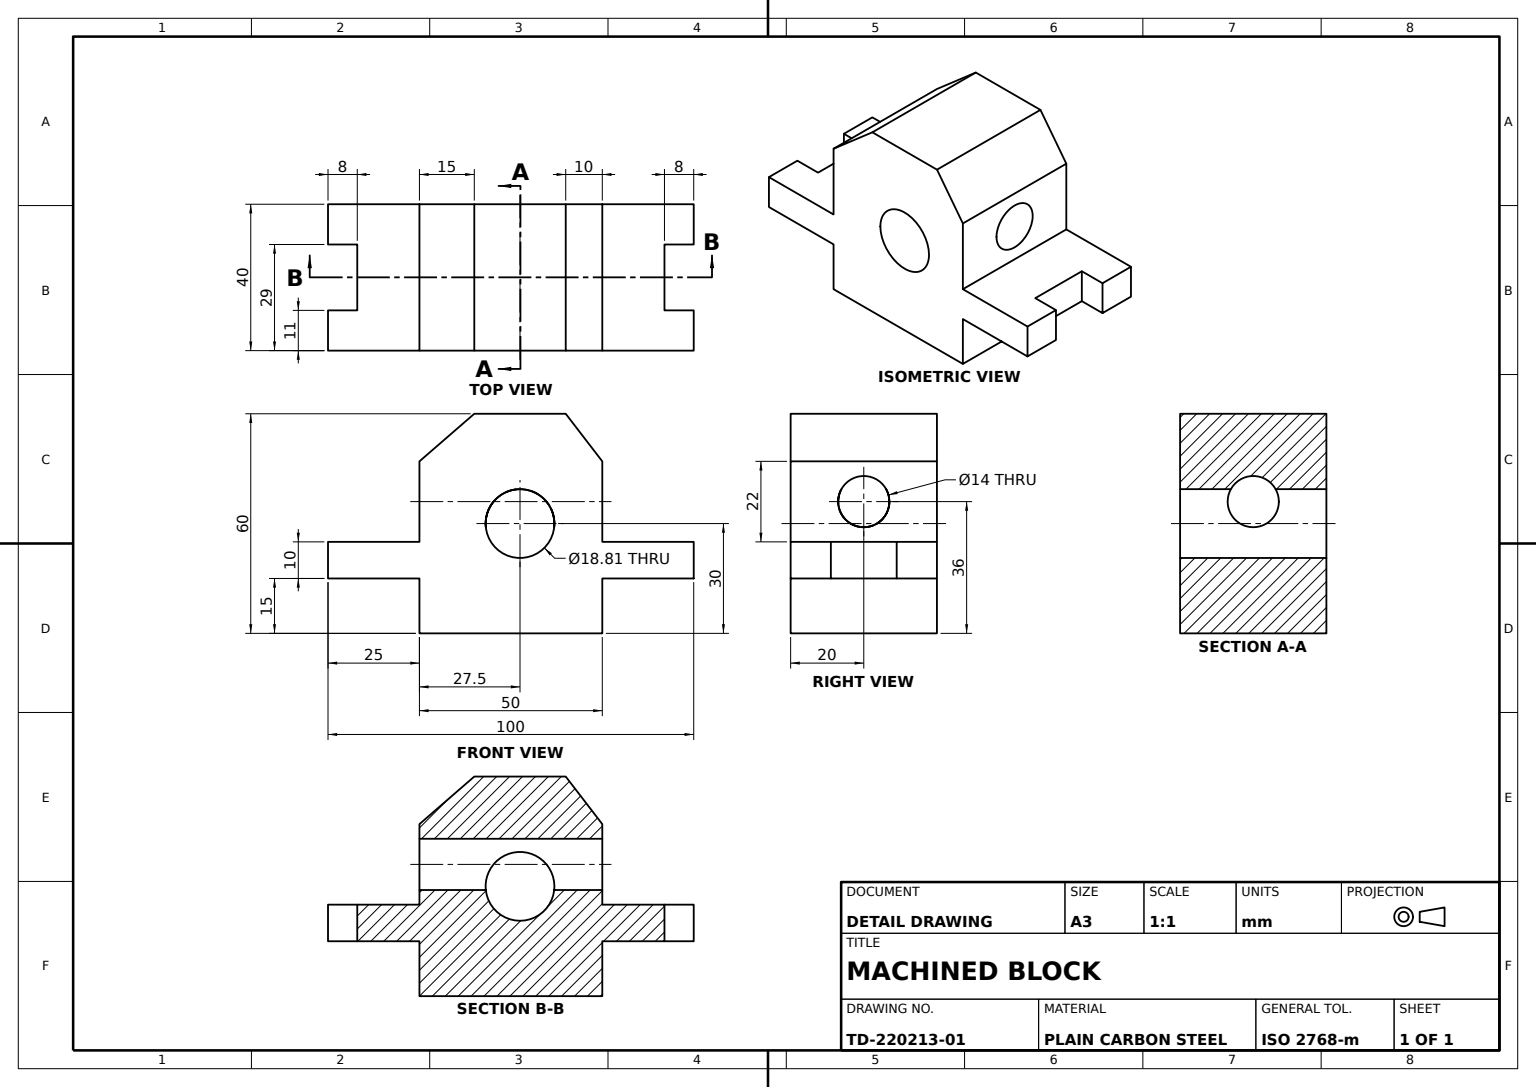
ISO-10303-21;
HEADER;
FILE_DESCRIPTION((''),'2;1');
FILE_NAME('','',(''),(''),'','','');
FILE_SCHEMA(('AUTOMOTIVE_DESIGN'));
ENDSEC;
DATA;
#1=APPLICATION_CONTEXT('');
#2=PRODUCT_CONTEXT('',#1,'mechanical');
#3=PRODUCT('','','',(#2));
#4=PRODUCT_DEFINITION_FORMATION('','',#3);
#5=PRODUCT_DEFINITION_CONTEXT('',#1,'design');
#6=PRODUCT_DEFINITION('','',#4,#5);
#7=PRODUCT_DEFINITION_SHAPE('','',#6);
#8=(LENGTH_UNIT()NAMED_UNIT(*)SI_UNIT(.MILLI.,.METRE.));
#9=(NAMED_UNIT(*)PLANE_ANGLE_UNIT()SI_UNIT($,.RADIAN.));
#10=(NAMED_UNIT(*)SI_UNIT($,.STERADIAN.)SOLID_ANGLE_UNIT());
#11=UNCERTAINTY_MEASURE_WITH_UNIT(LENGTH_MEASURE(1.E-05),#8,'distance_accuracy_value','');
#12=(GEOMETRIC_REPRESENTATION_CONTEXT(3)GLOBAL_UNCERTAINTY_ASSIGNED_CONTEXT((#11))GLOBAL_UNIT_ASSIGNED_CONTEXT((#8,#9,#10))REPRESENTATION_CONTEXT('',''));
#13=CARTESIAN_POINT('',(50.,36.,27.));
#14=VERTEX_POINT('',#13);
#15=CARTESIAN_POINT('',(50.,36.,13.));
#16=VERTEX_POINT('',#15);
#17=CARTESIAN_POINT('',(50.,36.,20.));
#18=DIRECTION('',(1.,0.,0.));
#19=DIRECTION('',(0.,0.,-1.));
#20=AXIS2_PLACEMENT_3D('',#17,#18,#19);
#21=CIRCLE('',#20,7.);
#22=EDGE_CURVE('',#14,#16,#21,.T.);
#23=ORIENTED_EDGE('',*,*,#22,.F.);
#24=EDGE_CURVE('',#16,#14,#21,.T.);
#25=ORIENTED_EDGE('',*,*,#24,.F.);
#26=EDGE_LOOP('',(#23,#25));
#27=FACE_BOUND('',#26,.T.);
#28=CARTESIAN_POINT('',(50.,25.,0.));
#29=VERTEX_POINT('',#28);
#30=CARTESIAN_POINT('',(50.,47.,0.));
#31=VERTEX_POINT('',#30);
#32=DIRECTION('',(0.,1.,0.));
#33=VECTOR('',#32,1000.);
#34=LINE('',#28,#33);
#35=EDGE_CURVE('',#29,#31,#34,.T.);
#36=ORIENTED_EDGE('',*,*,#35,.T.);
#37=CARTESIAN_POINT('',(50.,47.,40.));
#38=VERTEX_POINT('',#37);
#39=VECTOR('',#19,1000.);
#40=LINE('',#37,#39);
#41=EDGE_CURVE('',#38,#31,#40,.T.);
#42=ORIENTED_EDGE('',*,*,#41,.F.);
#43=CARTESIAN_POINT('',(50.,25.,40.));
#44=VERTEX_POINT('',#43);
#45=LINE('',#43,#33);
#46=EDGE_CURVE('',#44,#38,#45,.T.);
#47=ORIENTED_EDGE('',*,*,#46,.F.);
#48=LINE('',#43,#39);
#49=EDGE_CURVE('',#44,#29,#48,.T.);
#50=ORIENTED_EDGE('',*,*,#49,.T.);
#51=EDGE_LOOP('',(#36,#42,#47,#50));
#52=FACE_OUTER_BOUND('',#51,.T.);
#53=DIRECTION('',(-1.,0.,0.));
#54=DIRECTION('',(0.,0.,1.));
#55=AXIS2_PLACEMENT_3D('',#43,#53,#54);
#56=PLANE('',#55);
#57=ADVANCED_FACE('',(#27,#52),#56,.F.);
#58=CARTESIAN_POINT('',(50.,15.,40.));
#59=VERTEX_POINT('',#58);
#60=CARTESIAN_POINT('',(50.,15.,0.));
#61=VERTEX_POINT('',#60);
#62=LINE('',#58,#39);
#63=EDGE_CURVE('',#59,#61,#62,.T.);
#64=ORIENTED_EDGE('',*,*,#63,.F.);
#65=CARTESIAN_POINT('',(50.,0.,40.));
#66=VERTEX_POINT('',#65);
#67=LINE('',#65,#33);
#68=EDGE_CURVE('',#66,#59,#67,.T.);
#69=ORIENTED_EDGE('',*,*,#68,.F.);
#70=CARTESIAN_POINT('',(50.,0.,0.));
#71=VERTEX_POINT('',#70);
#72=LINE('',#65,#39);
#73=EDGE_CURVE('',#66,#71,#72,.T.);
#74=ORIENTED_EDGE('',*,*,#73,.T.);
#75=LINE('',#70,#33);
#76=EDGE_CURVE('',#71,#61,#75,.T.);
#77=ORIENTED_EDGE('',*,*,#76,.T.);
#78=EDGE_LOOP('',(#64,#69,#74,#77));
#79=FACE_OUTER_BOUND('',#78,.T.);
#80=AXIS2_PLACEMENT_3D('',#65,#53,#54);
#81=PLANE('',#80);
#82=ADVANCED_FACE('',(#79),#81,.F.);
#83=CARTESIAN_POINT('',(67.,25.,11.));
#84=VERTEX_POINT('',#83);
#85=CARTESIAN_POINT('',(67.,25.,29.));
#86=VERTEX_POINT('',#85);
#87=VECTOR('',#54,1000.);
#88=LINE('',#83,#87);
#89=EDGE_CURVE('',#84,#86,#88,.T.);
#90=ORIENTED_EDGE('',*,*,#89,.F.);
#91=CARTESIAN_POINT('',(75.,25.,11.));
#92=VERTEX_POINT('',#91);
#93=VECTOR('',#53,1000.);
#94=LINE('',#91,#93);
#95=EDGE_CURVE('',#92,#84,#94,.T.);
#96=ORIENTED_EDGE('',*,*,#95,.F.);
#97=CARTESIAN_POINT('',(75.,25.,0.));
#98=VERTEX_POINT('',#97);
#99=CARTESIAN_POINT('',(75.,25.,40.));
#100=LINE('',#99,#39);
#101=EDGE_CURVE('',#92,#98,#100,.T.);
#102=ORIENTED_EDGE('',*,*,#101,.T.);
#103=LINE('',#97,#93);
#104=EDGE_CURVE('',#98,#29,#103,.T.);
#105=ORIENTED_EDGE('',*,*,#104,.T.);
#106=ORIENTED_EDGE('',*,*,#49,.F.);
#107=VERTEX_POINT('',#99);
#108=LINE('',#99,#93);
#109=EDGE_CURVE('',#107,#44,#108,.T.);
#110=ORIENTED_EDGE('',*,*,#109,.F.);
#111=CARTESIAN_POINT('',(75.,25.,29.));
#112=VERTEX_POINT('',#111);
#113=EDGE_CURVE('',#107,#112,#100,.T.);
#114=ORIENTED_EDGE('',*,*,#113,.T.);
#115=VECTOR('',#18,1000.);
#116=LINE('',#85,#115);
#117=EDGE_CURVE('',#86,#112,#116,.T.);
#118=ORIENTED_EDGE('',*,*,#117,.F.);
#119=EDGE_LOOP('',(#90,#96,#102,#105,#106,#110,#114,#118));
#120=FACE_OUTER_BOUND('',#119,.T.);
#121=DIRECTION('',(0.,-1.,0.));
#122=AXIS2_PLACEMENT_3D('',#99,#121,#19);
#123=PLANE('',#122);
#124=ADVANCED_FACE('',(#120),#123,.F.);
#125=CARTESIAN_POINT('',(75.,15.,29.));
#126=VERTEX_POINT('',#125);
#127=CARTESIAN_POINT('',(75.,-15.,29.));
#128=LINE('',#127,#33);
#129=EDGE_CURVE('',#126,#112,#128,.T.);
#130=ORIENTED_EDGE('',*,*,#129,.T.);
#131=ORIENTED_EDGE('',*,*,#113,.F.);
#132=CARTESIAN_POINT('',(75.,15.,40.));
#133=VERTEX_POINT('',#132);
#134=LINE('',#132,#33);
#135=EDGE_CURVE('',#133,#107,#134,.T.);
#136=ORIENTED_EDGE('',*,*,#135,.F.);
#137=LINE('',#132,#39);
#138=EDGE_CURVE('',#133,#126,#137,.T.);
#139=ORIENTED_EDGE('',*,*,#138,.T.);
#140=EDGE_LOOP('',(#130,#131,#136,#139));
#141=FACE_OUTER_BOUND('',#140,.T.);
#142=AXIS2_PLACEMENT_3D('',#132,#53,#54);
#143=PLANE('',#142);
#144=ADVANCED_FACE('',(#141),#143,.F.);
#145=ORIENTED_EDGE('',*,*,#41,.T.);
#146=CARTESIAN_POINT('',(40.,60.,0.));
#147=VERTEX_POINT('',#146);
#148=DIRECTION('',(0.609710761,-0.792623989,0.));
#149=VECTOR('',#148,1000.);
#150=LINE('',#146,#149);
#151=EDGE_CURVE('',#147,#31,#150,.T.);
#152=ORIENTED_EDGE('',*,*,#151,.F.);
#153=CARTESIAN_POINT('',(40.,60.,40.));
#154=VERTEX_POINT('',#153);
#155=LINE('',#153,#39);
#156=EDGE_CURVE('',#154,#147,#155,.T.);
#157=ORIENTED_EDGE('',*,*,#156,.F.);
#158=LINE('',#153,#149);
#159=EDGE_CURVE('',#154,#38,#158,.T.);
#160=ORIENTED_EDGE('',*,*,#159,.T.);
#161=EDGE_LOOP('',(#145,#152,#157,#160));
#162=FACE_OUTER_BOUND('',#161,.T.);
#163=DIRECTION('',(0.792623989,0.609710761,0.));
#164=DIRECTION('',(-0.609710761,0.792623989,0.));
#165=AXIS2_PLACEMENT_3D('',#153,#163,#164);
#166=PLANE('',#165);
#167=ADVANCED_FACE('',(#162),#166,.T.);
#168=CARTESIAN_POINT('',(0.,36.,27.));
#169=VERTEX_POINT('',#168);
#170=CARTESIAN_POINT('',(0.,36.,13.));
#171=VERTEX_POINT('',#170);
#172=CARTESIAN_POINT('',(0.,36.,20.));
#173=AXIS2_PLACEMENT_3D('',#172,#53,#54);
#174=CIRCLE('',#173,7.);
#175=EDGE_CURVE('',#169,#171,#174,.T.);
#176=ORIENTED_EDGE('',*,*,#175,.F.);
#177=EDGE_CURVE('',#171,#169,#174,.T.);
#178=ORIENTED_EDGE('',*,*,#177,.F.);
#179=EDGE_LOOP('',(#176,#178));
#180=FACE_BOUND('',#179,.T.);
#181=CARTESIAN_POINT('',(0.,25.,0.));
#182=VERTEX_POINT('',#181);
#183=CARTESIAN_POINT('',(0.,47.,0.));
#184=VERTEX_POINT('',#183);
#185=LINE('',#181,#33);
#186=EDGE_CURVE('',#182,#184,#185,.T.);
#187=ORIENTED_EDGE('',*,*,#186,.F.);
#188=CARTESIAN_POINT('',(0.,25.,40.));
#189=VERTEX_POINT('',#188);
#190=LINE('',#188,#39);
#191=EDGE_CURVE('',#189,#182,#190,.T.);
#192=ORIENTED_EDGE('',*,*,#191,.F.);
#193=CARTESIAN_POINT('',(0.,47.,40.));
#194=VERTEX_POINT('',#193);
#195=LINE('',#188,#33);
#196=EDGE_CURVE('',#189,#194,#195,.T.);
#197=ORIENTED_EDGE('',*,*,#196,.T.);
#198=LINE('',#193,#39);
#199=EDGE_CURVE('',#194,#184,#198,.T.);
#200=ORIENTED_EDGE('',*,*,#199,.T.);
#201=EDGE_LOOP('',(#187,#192,#197,#200));
#202=FACE_OUTER_BOUND('',#201,.T.);
#203=AXIS2_PLACEMENT_3D('',#188,#53,#54);
#204=PLANE('',#203);
#205=ADVANCED_FACE('',(#180,#202),#204,.T.);
#206=CARTESIAN_POINT('',(75.,15.,11.));
#207=VERTEX_POINT('',#206);
#208=CARTESIAN_POINT('',(75.,-15.,11.));
#209=LINE('',#208,#33);
#210=EDGE_CURVE('',#207,#92,#209,.T.);
#211=ORIENTED_EDGE('',*,*,#210,.T.);
#212=ORIENTED_EDGE('',*,*,#95,.T.);
#213=CARTESIAN_POINT('',(67.,15.,11.));
#214=VERTEX_POINT('',#213);
#215=CARTESIAN_POINT('',(67.,-15.,11.));
#216=LINE('',#215,#33);
#217=EDGE_CURVE('',#214,#84,#216,.T.);
#218=ORIENTED_EDGE('',*,*,#217,.F.);
#219=CARTESIAN_POINT('',(50.,15.,11.));
#220=LINE('',#219,#93);
#221=EDGE_CURVE('',#207,#214,#220,.T.);
#222=ORIENTED_EDGE('',*,*,#221,.F.);
#223=EDGE_LOOP('',(#211,#212,#218,#222));
#224=FACE_OUTER_BOUND('',#223,.T.);
#225=AXIS2_PLACEMENT_3D('',#208,#19,#53);
#226=PLANE('',#225);
#227=ADVANCED_FACE('',(#224),#226,.F.);
#228=CARTESIAN_POINT('',(36.903768,30.,40.));
#229=VERTEX_POINT('',#228);
#230=CARTESIAN_POINT('',(18.096232,30.,40.));
#231=VERTEX_POINT('',#230);
#232=CARTESIAN_POINT('',(27.5,30.,40.));
#233=AXIS2_PLACEMENT_3D('',#232,#54,#18);
#234=CIRCLE('',#233,9.403768);
#235=EDGE_CURVE('',#229,#231,#234,.T.);
#236=ORIENTED_EDGE('',*,*,#235,.T.);
#237=CARTESIAN_POINT('',(18.096232,30.,23.605551));
#238=VERTEX_POINT('',#237);
#239=CARTESIAN_POINT('',(18.096232,30.,0.));
#240=LINE('',#239,#87);
#241=EDGE_CURVE('',#238,#231,#240,.T.);
#242=ORIENTED_EDGE('',*,*,#241,.F.);
#243=CARTESIAN_POINT('',(20.259084,36.,27.));
#244=VERTEX_POINT('',#243);
#245=CARTESIAN_POINT('',(18.096232,30.33094,24.156269));
#246=CARTESIAN_POINT('',(18.112771,30.730821,24.653008));
#247=CARTESIAN_POINT('',(18.20319,31.43388,25.315471));
#248=CARTESIAN_POINT('',(18.244042,31.681225,25.517877));
#249=CARTESIAN_POINT('',(18.351805,32.193127,25.88273));
#250=CARTESIAN_POINT('',(18.41881,32.458633,26.046052));
#251=CARTESIAN_POINT('',(18.585264,33.00672,26.335321));
#252=CARTESIAN_POINT('',(18.685614,33.290821,26.461416));
#253=CARTESIAN_POINT('',(18.916067,33.852142,26.669052));
#254=CARTESIAN_POINT('',(19.04675,34.131839,26.752122));
#255=CARTESIAN_POINT('',(19.341329,34.68675,26.881609));
#256=CARTESIAN_POINT('',(19.506599,34.963767,26.928055));
#257=CARTESIAN_POINT('',(19.862851,35.496125,26.986976));
#258=CARTESIAN_POINT('',(20.054302,35.752864,27.));
#259=B_SPLINE_CURVE_WITH_KNOTS('',3,(#237,#245,#246,#247,#248,#249,#250,#251,#252,#253,#254,#255,#256,#257,#258,#243),.UNSPECIFIED.,.F.,.F.,(4,2,2,2,2,2,2,4),(0.039471244,0.041386587,0.042344259,0.04330193,0.044259602,0.045217273,0.046174945,0.047132616),.UNSPECIFIED.);
#260=EDGE_CURVE('',#238,#244,#259,.T.);
#261=ORIENTED_EDGE('',*,*,#260,.T.);
#262=CARTESIAN_POINT('',(34.740916,36.,27.));
#263=VERTEX_POINT('',#262);
#264=CARTESIAN_POINT('',(20.480719,36.267473,27.));
#265=CARTESIAN_POINT('',(20.719708,36.52524,26.984471));
#266=CARTESIAN_POINT('',(21.21874,37.006918,26.931437));
#267=CARTESIAN_POINT('',(21.478974,37.231549,26.894131));
#268=CARTESIAN_POINT('',(22.020747,37.650218,26.806066));
#269=CARTESIAN_POINT('',(22.302285,37.844249,26.75527));
#270=CARTESIAN_POINT('',(22.88751,38.202037,26.647251));
#271=CARTESIAN_POINT('',(23.192469,38.366202,26.589796));
#272=CARTESIAN_POINT('',(24.122486,38.80298,26.421886));
#273=CARTESIAN_POINT('',(24.767744,39.024604,26.315107));
#274=CARTESIAN_POINT('',(25.779513,39.2515,26.199593));
#275=CARTESIAN_POINT('',(26.124787,39.309074,26.168622));
#276=CARTESIAN_POINT('',(26.811152,39.384858,26.127365));
#277=CARTESIAN_POINT('',(27.154616,39.403708,26.116761));
#278=CARTESIAN_POINT('',(27.842109,39.403828,26.116695));
#279=CARTESIAN_POINT('',(28.186138,39.385098,26.127233));
#280=CARTESIAN_POINT('',(28.874765,39.309182,26.168564));
#281=CARTESIAN_POINT('',(29.220402,39.25149,26.199595));
#282=CARTESIAN_POINT('',(30.230191,39.025125,26.314847));
#283=CARTESIAN_POINT('',(30.876899,38.803521,26.421746));
#284=CARTESIAN_POINT('',(31.812065,38.363946,26.59063));
#285=CARTESIAN_POINT('',(32.114887,38.200631,26.647697));
#286=CARTESIAN_POINT('',(32.697705,37.844196,26.755264));
#287=CARTESIAN_POINT('',(32.978731,37.650596,26.805976));
#288=CARTESIAN_POINT('',(33.520654,37.231862,26.894076));
#289=CARTESIAN_POINT('',(33.781553,37.006739,26.931506));
#290=CARTESIAN_POINT('',(34.282921,36.522598,26.984712));
#291=CARTESIAN_POINT('',(34.520014,36.266589,27.));
#292=B_SPLINE_CURVE_WITH_KNOTS('',3,(#243,#264,#265,#266,#267,#268,#269,#270,#271,#272,#273,#274,#275,#276,#277,#278,#279,#280,#281,#282,#283,#284,#285,#286,#287,#288,#289,#290,#291,#262),.UNSPECIFIED.,.F.,.F.,(4,2,2,2,2,2,2,2,2,2,2,2,2,2,4),(0.047132616,0.048169096,0.049205576,0.050242055,0.051278535,0.053351494,0.054387974,0.055424454,0.056460933,0.057497413,0.059570372,0.060606852,0.061643332,0.062679811,0.063716291),.UNSPECIFIED.);
#293=EDGE_CURVE('',#244,#263,#292,.T.);
#294=ORIENTED_EDGE('',*,*,#293,.T.);
#295=CARTESIAN_POINT('',(36.903768,30.,23.605551));
#296=VERTEX_POINT('',#295);
#297=CARTESIAN_POINT('',(34.944818,35.753927,27.));
#298=CARTESIAN_POINT('',(35.13573,35.49806,26.987092));
#299=CARTESIAN_POINT('',(35.491449,34.966868,26.928495));
#300=CARTESIAN_POINT('',(35.656946,34.689708,26.882145));
#301=CARTESIAN_POINT('',(35.951157,34.13607,26.753262));
#302=CARTESIAN_POINT('',(36.081383,33.857661,26.670728));
#303=CARTESIAN_POINT('',(36.310783,33.30027,26.465267));
#304=CARTESIAN_POINT('',(36.410251,33.020261,26.341834));
#305=CARTESIAN_POINT('',(36.663446,32.190171,25.905593));
#306=CARTESIAN_POINT('',(36.765551,31.674666,25.541364));
#307=CARTESIAN_POINT('',(36.886889,30.735707,24.658589));
#308=CARTESIAN_POINT('',(36.903768,30.332441,24.158766));
#309=B_SPLINE_CURVE_WITH_KNOTS('',3,(#262,#297,#298,#299,#300,#301,#302,#303,#304,#305,#306,#307,#308,#295),.UNSPECIFIED.,.F.,.F.,(4,2,2,2,2,2,4),(0.063716291,0.064673006,0.065629721,0.066586437,0.067543152,0.069456582,0.071370013),.UNSPECIFIED.);
#310=EDGE_CURVE('',#263,#296,#309,.T.);
#311=ORIENTED_EDGE('',*,*,#310,.T.);
#312=CARTESIAN_POINT('',(36.903768,30.,0.));
#313=LINE('',#312,#87);
#314=EDGE_CURVE('',#296,#229,#313,.T.);
#315=ORIENTED_EDGE('',*,*,#314,.T.);
#316=EDGE_LOOP('',(#236,#242,#261,#294,#311,#315));
#317=FACE_OUTER_BOUND('',#316,.T.);
#318=CARTESIAN_POINT('',(27.5,30.,0.));
#319=AXIS2_PLACEMENT_3D('',#318,#54,#18);
#320=CYLINDRICAL_SURFACE('',#319,9.403768);
#321=ADVANCED_FACE('',(#317),#320,.F.);
#322=ORIENTED_EDGE('',*,*,#175,.T.);
#323=CARTESIAN_POINT('',(20.259084,36.,13.));
#324=VERTEX_POINT('',#323);
#325=CARTESIAN_POINT('',(-25.,36.,13.));
#326=LINE('',#325,#115);
#327=EDGE_CURVE('',#171,#324,#326,.T.);
#328=ORIENTED_EDGE('',*,*,#327,.T.);
#329=CARTESIAN_POINT('',(34.740916,36.,13.));
#330=VERTEX_POINT('',#329);
#331=CARTESIAN_POINT('',(34.519378,36.267356,13.));
#332=CARTESIAN_POINT('',(34.28068,36.524858,13.015491));
#333=CARTESIAN_POINT('',(33.78109,37.007089,13.068578));
#334=CARTESIAN_POINT('',(33.520697,37.231823,13.105918));
#335=CARTESIAN_POINT('',(32.97889,37.650479,13.193997));
#336=CARTESIAN_POINT('',(32.697475,37.844393,13.244775));
#337=CARTESIAN_POINT('',(32.112829,38.201833,13.352686));
#338=CARTESIAN_POINT('',(31.807926,38.366012,13.410132));
#339=CARTESIAN_POINT('',(30.877033,38.803215,13.578202));
#340=CARTESIAN_POINT('',(30.231849,39.02465,13.68492));
#341=CARTESIAN_POINT('',(29.221588,39.251276,13.800291));
#342=CARTESIAN_POINT('',(28.875899,39.308994,13.831335));
#343=CARTESIAN_POINT('',(28.18841,39.384911,13.872664));
#344=CARTESIAN_POINT('',(27.50089,39.422562,13.893844));
#345=CARTESIAN_POINT('',(26.813307,39.385039,13.872735));
#346=CARTESIAN_POINT('',(26.125694,39.309231,13.831463));
#347=CARTESIAN_POINT('',(25.780035,39.251585,13.800453));
#348=CARTESIAN_POINT('',(24.769182,39.024991,13.685084));
#349=CARTESIAN_POINT('',(24.122632,38.803272,13.578166));
#350=CARTESIAN_POINT('',(23.188639,38.364291,13.409499));
#351=CARTESIAN_POINT('',(22.884958,38.200553,13.352273));
#352=CARTESIAN_POINT('',(22.301801,37.843877,13.244645));
#353=CARTESIAN_POINT('',(22.020795,37.650247,13.193944));
#354=CARTESIAN_POINT('',(21.479235,37.23176,13.105909));
#355=CARTESIAN_POINT('',(21.218681,37.006913,13.068537));
#356=CARTESIAN_POINT('',(20.718276,36.523804,13.015397));
#357=CARTESIAN_POINT('',(20.480146,36.266781,13.));
#358=B_SPLINE_CURVE_WITH_KNOTS('',3,(#329,#331,#332,#333,#334,#335,#336,#337,#338,#339,#340,#341,#342,#343,#344,#345,#346,#347,#348,#349,#350,#351,#352,#353,#354,#355,#356,#357,#323),.UNSPECIFIED.,.F.,.F.,(4,2,2,2,2,2,2,1,2,2,2,2,2,2,4),(0.007664159,0.0087021,0.009740041,0.010777982,0.011815923,0.013891805,0.014929745,0.015967686,0.017005627,0.018043568,0.02011945,0.02115739,0.022195331,0.023233272,0.024271213),.UNSPECIFIED.);
#359=EDGE_CURVE('',#330,#324,#358,.T.);
#360=ORIENTED_EDGE('',*,*,#359,.F.);
#361=EDGE_CURVE('',#330,#16,#326,.T.);
#362=ORIENTED_EDGE('',*,*,#361,.T.);
#363=ORIENTED_EDGE('',*,*,#24,.T.);
#364=CARTESIAN_POINT('',(-25.,36.,27.));
#365=LINE('',#364,#115);
#366=EDGE_CURVE('',#263,#14,#365,.T.);
#367=ORIENTED_EDGE('',*,*,#366,.F.);
#368=ORIENTED_EDGE('',*,*,#293,.F.);
#369=EDGE_CURVE('',#169,#244,#365,.T.);
#370=ORIENTED_EDGE('',*,*,#369,.F.);
#371=EDGE_LOOP('',(#322,#328,#360,#362,#363,#367,#368,#370));
#372=FACE_OUTER_BOUND('',#371,.T.);
#373=CARTESIAN_POINT('',(-25.,36.,20.));
#374=AXIS2_PLACEMENT_3D('',#373,#18,#19);
#375=CYLINDRICAL_SURFACE('',#374,7.);
#376=ADVANCED_FACE('',(#372),#375,.F.);
#377=CARTESIAN_POINT('',(-17.,15.,29.));
#378=VERTEX_POINT('',#377);
#379=CARTESIAN_POINT('',(-17.,25.,29.));
#380=VERTEX_POINT('',#379);
#381=CARTESIAN_POINT('',(-17.,-15.,29.));
#382=LINE('',#381,#33);
#383=EDGE_CURVE('',#378,#380,#382,.T.);
#384=ORIENTED_EDGE('',*,*,#383,.T.);
#385=CARTESIAN_POINT('',(-17.,25.,11.));
#386=VERTEX_POINT('',#385);
#387=LINE('',#385,#39);
#388=EDGE_CURVE('',#380,#386,#387,.T.);
#389=ORIENTED_EDGE('',*,*,#388,.T.);
#390=CARTESIAN_POINT('',(-17.,15.,11.));
#391=VERTEX_POINT('',#390);
#392=CARTESIAN_POINT('',(-17.,-15.,11.));
#393=LINE('',#392,#33);
#394=EDGE_CURVE('',#391,#386,#393,.T.);
#395=ORIENTED_EDGE('',*,*,#394,.F.);
#396=CARTESIAN_POINT('',(-17.,15.,40.));
#397=LINE('',#396,#87);
#398=EDGE_CURVE('',#391,#378,#397,.T.);
#399=ORIENTED_EDGE('',*,*,#398,.T.);
#400=EDGE_LOOP('',(#384,#389,#395,#399));
#401=FACE_OUTER_BOUND('',#400,.T.);
#402=AXIS2_PLACEMENT_3D('',#392,#18,#19);
#403=PLANE('',#402);
#404=ADVANCED_FACE('',(#401),#403,.F.);
#405=CARTESIAN_POINT('',(-25.,15.,40.));
#406=VERTEX_POINT('',#405);
#407=CARTESIAN_POINT('',(-25.,15.,29.));
#408=VERTEX_POINT('',#407);
#409=LINE('',#405,#39);
#410=EDGE_CURVE('',#406,#408,#409,.T.);
#411=ORIENTED_EDGE('',*,*,#410,.F.);
#412=CARTESIAN_POINT('',(-25.,25.,40.));
#413=VERTEX_POINT('',#412);
#414=LINE('',#405,#33);
#415=EDGE_CURVE('',#406,#413,#414,.T.);
#416=ORIENTED_EDGE('',*,*,#415,.T.);
#417=CARTESIAN_POINT('',(-25.,25.,29.));
#418=VERTEX_POINT('',#417);
#419=LINE('',#412,#39);
#420=EDGE_CURVE('',#413,#418,#419,.T.);
#421=ORIENTED_EDGE('',*,*,#420,.T.);
#422=CARTESIAN_POINT('',(-25.,-15.,29.));
#423=LINE('',#422,#33);
#424=EDGE_CURVE('',#408,#418,#423,.T.);
#425=ORIENTED_EDGE('',*,*,#424,.F.);
#426=EDGE_LOOP('',(#411,#416,#421,#425));
#427=FACE_OUTER_BOUND('',#426,.T.);
#428=AXIS2_PLACEMENT_3D('',#405,#53,#54);
#429=PLANE('',#428);
#430=ADVANCED_FACE('',(#427),#429,.T.);
#431=CARTESIAN_POINT('',(-25.,15.,0.));
#432=VERTEX_POINT('',#431);
#433=CARTESIAN_POINT('',(-25.,25.,0.));
#434=VERTEX_POINT('',#433);
#435=LINE('',#431,#33);
#436=EDGE_CURVE('',#432,#434,#435,.T.);
#437=ORIENTED_EDGE('',*,*,#436,.F.);
#438=CARTESIAN_POINT('',(-25.,15.,11.));
#439=VERTEX_POINT('',#438);
#440=EDGE_CURVE('',#439,#432,#409,.T.);
#441=ORIENTED_EDGE('',*,*,#440,.F.);
#442=CARTESIAN_POINT('',(-25.,25.,11.));
#443=VERTEX_POINT('',#442);
#444=CARTESIAN_POINT('',(-25.,-15.,11.));
#445=LINE('',#444,#33);
#446=EDGE_CURVE('',#439,#443,#445,.T.);
#447=ORIENTED_EDGE('',*,*,#446,.T.);
#448=EDGE_CURVE('',#443,#434,#419,.T.);
#449=ORIENTED_EDGE('',*,*,#448,.T.);
#450=EDGE_LOOP('',(#437,#441,#447,#449));
#451=FACE_OUTER_BOUND('',#450,.T.);
#452=ADVANCED_FACE('',(#451),#429,.T.);
#453=ORIENTED_EDGE('',*,*,#260,.F.);
#454=CARTESIAN_POINT('',(18.096232,30.,16.394449));
#455=VERTEX_POINT('',#454);
#456=CARTESIAN_POINT('',(18.096232,29.836753,16.666108));
#457=CARTESIAN_POINT('',(18.100474,29.691436,16.950217));
#458=CARTESIAN_POINT('',(18.111914,29.443088,17.528956));
#459=CARTESIAN_POINT('',(18.11912,29.338868,17.825458));
#460=CARTESIAN_POINT('',(18.132515,29.17041,18.432829));
#461=CARTESIAN_POINT('',(18.13873,29.105967,18.746102));
#462=CARTESIAN_POINT('',(18.147234,29.021,19.372687));
#463=CARTESIAN_POINT('',(18.149554,28.999988,19.68631));
#464=CARTESIAN_POINT('',(18.149552,29.000012,20.314207));
#465=CARTESIAN_POINT('',(18.147228,29.021044,20.62848));
#466=CARTESIAN_POINT('',(18.138668,29.106597,21.257697));
#467=CARTESIAN_POINT('',(18.13248,29.170823,21.568801));
#468=CARTESIAN_POINT('',(18.119119,29.338908,22.174547));
#469=CARTESIAN_POINT('',(18.11192,29.44297,22.470751));
#470=CARTESIAN_POINT('',(18.100473,29.691435,23.049798));
#471=CARTESIAN_POINT('',(18.096232,29.837241,23.334703));
#472=B_SPLINE_CURVE_WITH_KNOTS('',3,(#454,#456,#457,#458,#459,#460,#461,#462,#463,#464,#465,#466,#467,#468,#469,#470,#471,#237),.UNSPECIFIED.,.F.,.F.,(4,2,2,2,2,2,2,2,4),(0.031935379,0.032877362,0.033819345,0.034761328,0.035703311,0.036645295,0.037587278,0.038529261,0.039471244),.UNSPECIFIED.);
#473=EDGE_CURVE('',#455,#238,#472,.T.);
#474=ORIENTED_EDGE('',*,*,#473,.F.);
#475=CARTESIAN_POINT('',(20.055044,35.75376,13.));
#476=CARTESIAN_POINT('',(19.864196,35.497934,13.01293));
#477=CARTESIAN_POINT('',(19.508895,34.967397,13.071439));
#478=CARTESIAN_POINT('',(19.34334,34.690243,13.117732));
#479=CARTESIAN_POINT('',(18.90123,33.858302,13.311397));
#480=CARTESIAN_POINT('',(18.674568,33.298256,13.51211));
#481=CARTESIAN_POINT('',(18.336349,32.189576,14.09468));
#482=CARTESIAN_POINT('',(18.23437,31.674037,14.459238));
#483=CARTESIAN_POINT('',(18.143496,30.970852,15.120331));
#484=CARTESIAN_POINT('',(18.124149,30.751518,15.357168));
#485=CARTESIAN_POINT('',(18.100582,30.349705,15.855531));
#486=CARTESIAN_POINT('',(18.096232,30.166026,16.118164));
#487=B_SPLINE_CURVE_WITH_KNOTS('',3,(#323,#475,#476,#477,#478,#479,#480,#481,#482,#483,#484,#485,#486,#454),.UNSPECIFIED.,.F.,.F.,(4,2,2,2,2,2,4),(0.024271213,0.025229234,0.026187254,0.028103296,0.030019337,0.030977358,0.031935379),.UNSPECIFIED.);
#488=EDGE_CURVE('',#324,#455,#487,.T.);
#489=ORIENTED_EDGE('',*,*,#488,.F.);
#490=ORIENTED_EDGE('',*,*,#327,.F.);
#491=ORIENTED_EDGE('',*,*,#177,.T.);
#492=ORIENTED_EDGE('',*,*,#369,.T.);
#493=EDGE_LOOP('',(#453,#474,#489,#490,#491,#492));
#494=FACE_OUTER_BOUND('',#493,.T.);
#495=ADVANCED_FACE('',(#494),#375,.F.);
#496=CARTESIAN_POINT('',(67.,15.,29.));
#497=VERTEX_POINT('',#496);
#498=CARTESIAN_POINT('',(67.,-15.,29.));
#499=LINE('',#498,#33);
#500=EDGE_CURVE('',#497,#86,#499,.T.);
#501=ORIENTED_EDGE('',*,*,#500,.T.);
#502=ORIENTED_EDGE('',*,*,#117,.T.);
#503=ORIENTED_EDGE('',*,*,#129,.F.);
#504=CARTESIAN_POINT('',(50.,15.,29.));
#505=LINE('',#504,#115);
#506=EDGE_CURVE('',#497,#126,#505,.T.);
#507=ORIENTED_EDGE('',*,*,#506,.F.);
#508=EDGE_LOOP('',(#501,#502,#503,#507));
#509=FACE_OUTER_BOUND('',#508,.T.);
#510=AXIS2_PLACEMENT_3D('',#498,#54,#18);
#511=PLANE('',#510);
#512=ADVANCED_FACE('',(#509),#511,.F.);
#513=CARTESIAN_POINT('',(75.,15.,0.));
#514=VERTEX_POINT('',#513);
#515=LINE('',#513,#33);
#516=EDGE_CURVE('',#514,#98,#515,.T.);
#517=ORIENTED_EDGE('',*,*,#516,.T.);
#518=ORIENTED_EDGE('',*,*,#101,.F.);
#519=ORIENTED_EDGE('',*,*,#210,.F.);
#520=EDGE_CURVE('',#207,#514,#137,.T.);
#521=ORIENTED_EDGE('',*,*,#520,.T.);
#522=EDGE_LOOP('',(#517,#518,#519,#521));
#523=FACE_OUTER_BOUND('',#522,.T.);
#524=ADVANCED_FACE('',(#523),#143,.F.);
#525=ORIENTED_EDGE('',*,*,#488,.T.);
#526=VERTEX_POINT('',#239);
#527=EDGE_CURVE('',#526,#455,#240,.T.);
#528=ORIENTED_EDGE('',*,*,#527,.F.);
#529=VERTEX_POINT('',#312);
#530=CIRCLE('',#319,9.403768);
#531=EDGE_CURVE('',#529,#526,#530,.T.);
#532=ORIENTED_EDGE('',*,*,#531,.F.);
#533=CARTESIAN_POINT('',(36.903768,30.,16.394449));
#534=VERTEX_POINT('',#533);
#535=EDGE_CURVE('',#529,#534,#313,.T.);
#536=ORIENTED_EDGE('',*,*,#535,.T.);
#537=CARTESIAN_POINT('',(36.903768,30.333297,15.83981));
#538=CARTESIAN_POINT('',(36.886834,30.734674,15.343022));
#539=CARTESIAN_POINT('',(36.796628,31.434902,14.683737));
#540=CARTESIAN_POINT('',(36.755464,31.684009,14.479923));
#541=CARTESIAN_POINT('',(36.647345,32.19672,14.114927));
#542=CARTESIAN_POINT('',(36.580196,32.462248,13.951863));
#543=CARTESIAN_POINT('',(36.413809,33.009424,13.663431));
#544=CARTESIAN_POINT('',(36.313479,33.293255,13.537565));
#545=CARTESIAN_POINT('',(36.082821,33.854623,13.33015));
#546=CARTESIAN_POINT('',(35.952138,34.134074,13.247282));
#547=CARTESIAN_POINT('',(35.65793,34.688004,13.118173));
#548=CARTESIAN_POINT('',(35.492958,34.964477,13.071841));
#549=CARTESIAN_POINT('',(35.136712,35.49673,13.012983));
#550=CARTESIAN_POINT('',(34.945395,35.753231,13.));
#551=B_SPLINE_CURVE_WITH_KNOTS('',3,(#533,#537,#538,#539,#540,#541,#542,#543,#544,#545,#546,#547,#548,#549,#550,#329),.UNSPECIFIED.,.F.,.F.,(4,2,2,2,2,2,2,4),(0.,0.00191604,0.00287406,0.00383208,0.0047901,0.00574812,0.00670614,0.007664159),.UNSPECIFIED.);
#552=EDGE_CURVE('',#534,#330,#551,.T.);
#553=ORIENTED_EDGE('',*,*,#552,.T.);
#554=ORIENTED_EDGE('',*,*,#359,.T.);
#555=EDGE_LOOP('',(#525,#528,#532,#536,#553,#554));
#556=FACE_OUTER_BOUND('',#555,.T.);
#557=ADVANCED_FACE('',(#556),#320,.F.);
#558=CARTESIAN_POINT('',(0.,15.,29.));
#559=LINE('',#558,#93);
#560=EDGE_CURVE('',#378,#408,#559,.T.);
#561=ORIENTED_EDGE('',*,*,#560,.T.);
#562=ORIENTED_EDGE('',*,*,#424,.T.);
#563=LINE('',#379,#115);
#564=EDGE_CURVE('',#418,#380,#563,.T.);
#565=ORIENTED_EDGE('',*,*,#564,.T.);
#566=ORIENTED_EDGE('',*,*,#383,.F.);
#567=EDGE_LOOP('',(#561,#562,#565,#566));
#568=FACE_OUTER_BOUND('',#567,.T.);
#569=AXIS2_PLACEMENT_3D('',#381,#54,#18);
#570=PLANE('',#569);
#571=ADVANCED_FACE('',(#568),#570,.F.);
#572=ORIENTED_EDGE('',*,*,#235,.F.);
#573=EDGE_CURVE('',#231,#229,#234,.T.);
#574=ORIENTED_EDGE('',*,*,#573,.F.);
#575=EDGE_LOOP('',(#572,#574));
#576=FACE_BOUND('',#575,.T.);
#577=CARTESIAN_POINT('',(15.,60.,40.));
#578=VERTEX_POINT('',#577);
#579=LINE('',#577,#115);
#580=EDGE_CURVE('',#578,#154,#579,.T.);
#581=ORIENTED_EDGE('',*,*,#580,.F.);
#582=DIRECTION('',(0.755689083,0.654930538,0.));
#583=VECTOR('',#582,1000.);
#584=LINE('',#193,#583);
#585=EDGE_CURVE('',#194,#578,#584,.T.);
#586=ORIENTED_EDGE('',*,*,#585,.F.);
#587=ORIENTED_EDGE('',*,*,#196,.F.);
#588=LINE('',#412,#115);
#589=EDGE_CURVE('',#413,#189,#588,.T.);
#590=ORIENTED_EDGE('',*,*,#589,.F.);
#591=ORIENTED_EDGE('',*,*,#415,.F.);
#592=CARTESIAN_POINT('',(0.,15.,40.));
#593=VERTEX_POINT('',#592);
#594=LINE('',#592,#93);
#595=EDGE_CURVE('',#593,#406,#594,.T.);
#596=ORIENTED_EDGE('',*,*,#595,.F.);
#597=CARTESIAN_POINT('',(0.,0.,40.));
#598=VERTEX_POINT('',#597);
#599=LINE('',#597,#33);
#600=EDGE_CURVE('',#598,#593,#599,.T.);
#601=ORIENTED_EDGE('',*,*,#600,.F.);
#602=LINE('',#597,#115);
#603=EDGE_CURVE('',#598,#66,#602,.T.);
#604=ORIENTED_EDGE('',*,*,#603,.T.);
#605=ORIENTED_EDGE('',*,*,#68,.T.);
#606=LINE('',#58,#115);
#607=EDGE_CURVE('',#59,#133,#606,.T.);
#608=ORIENTED_EDGE('',*,*,#607,.T.);
#609=ORIENTED_EDGE('',*,*,#135,.T.);
#610=ORIENTED_EDGE('',*,*,#109,.T.);
#611=ORIENTED_EDGE('',*,*,#46,.T.);
#612=ORIENTED_EDGE('',*,*,#159,.F.);
#613=EDGE_LOOP('',(#581,#586,#587,#590,#591,#596,#601,#604,#605,#608,#609,#610,#611,#612));
#614=FACE_OUTER_BOUND('',#613,.T.);
#615=AXIS2_PLACEMENT_3D('',#597,#54,#18);
#616=PLANE('',#615);
#617=ADVANCED_FACE('',(#576,#614),#616,.T.);
#618=CARTESIAN_POINT('',(0.,15.,11.));
#619=LINE('',#618,#115);
#620=EDGE_CURVE('',#439,#391,#619,.T.);
#621=ORIENTED_EDGE('',*,*,#620,.T.);
#622=ORIENTED_EDGE('',*,*,#394,.T.);
#623=LINE('',#442,#93);
#624=EDGE_CURVE('',#386,#443,#623,.T.);
#625=ORIENTED_EDGE('',*,*,#624,.T.);
#626=ORIENTED_EDGE('',*,*,#446,.F.);
#627=EDGE_LOOP('',(#621,#622,#625,#626));
#628=FACE_OUTER_BOUND('',#627,.T.);
#629=AXIS2_PLACEMENT_3D('',#444,#19,#53);
#630=PLANE('',#629);
#631=ADVANCED_FACE('',(#628),#630,.F.);
#632=ORIENTED_EDGE('',*,*,#199,.F.);
#633=ORIENTED_EDGE('',*,*,#585,.T.);
#634=CARTESIAN_POINT('',(15.,60.,0.));
#635=VERTEX_POINT('',#634);
#636=LINE('',#577,#39);
#637=EDGE_CURVE('',#578,#635,#636,.T.);
#638=ORIENTED_EDGE('',*,*,#637,.T.);
#639=LINE('',#183,#583);
#640=EDGE_CURVE('',#184,#635,#639,.T.);
#641=ORIENTED_EDGE('',*,*,#640,.F.);
#642=EDGE_LOOP('',(#632,#633,#638,#641));
#643=FACE_OUTER_BOUND('',#642,.T.);
#644=DIRECTION('',(-0.654930538,0.755689083,0.));
#645=DIRECTION('',(-0.755689083,-0.654930538,0.));
#646=AXIS2_PLACEMENT_3D('',#193,#644,#645);
#647=PLANE('',#646);
#648=ADVANCED_FACE('',(#643),#647,.T.);
#649=ORIENTED_EDGE('',*,*,#241,.T.);
#650=ORIENTED_EDGE('',*,*,#573,.T.);
#651=ORIENTED_EDGE('',*,*,#314,.F.);
#652=CARTESIAN_POINT('',(36.903768,29.836604,23.333644));
#653=CARTESIAN_POINT('',(36.899532,29.69164,23.050181));
#654=CARTESIAN_POINT('',(36.888104,29.443414,22.471879));
#655=CARTESIAN_POINT('',(36.8809,29.339144,22.175416));
#656=CARTESIAN_POINT('',(36.867496,29.170524,21.567705));
#657=CARTESIAN_POINT('',(36.861278,29.106051,21.254249));
#658=CARTESIAN_POINT('',(36.85278,29.021132,20.628551));
#659=CARTESIAN_POINT('',(36.850453,29.000054,20.315152));
#660=CARTESIAN_POINT('',(36.850441,28.999946,19.687269));
#661=CARTESIAN_POINT('',(36.852758,29.020911,19.372785));
#662=CARTESIAN_POINT('',(36.861323,29.106505,18.742694));
#663=CARTESIAN_POINT('',(36.867487,29.17047,18.43278));
#664=CARTESIAN_POINT('',(36.880835,29.33828,17.827411));
#665=CARTESIAN_POINT('',(36.888036,29.442233,17.531178));
#666=CARTESIAN_POINT('',(36.899503,29.690708,16.951685));
#667=CARTESIAN_POINT('',(36.903768,29.836406,16.666685));
#668=B_SPLINE_CURVE_WITH_KNOTS('',3,(#295,#652,#653,#654,#655,#656,#657,#658,#659,#660,#661,#662,#663,#664,#665,#666,#667,#533),.UNSPECIFIED.,.F.,.F.,(4,2,2,2,2,2,2,2,4),(0.071370013,0.072310472,0.073250932,0.074191392,0.075131851,0.076072311,0.07701277,0.07795323,0.07889369),.UNSPECIFIED.);
#669=EDGE_CURVE('',#296,#534,#668,.T.);
#670=ORIENTED_EDGE('',*,*,#669,.T.);
#671=ORIENTED_EDGE('',*,*,#535,.F.);
#672=EDGE_CURVE('',#526,#529,#530,.T.);
#673=ORIENTED_EDGE('',*,*,#672,.F.);
#674=ORIENTED_EDGE('',*,*,#527,.T.);
#675=ORIENTED_EDGE('',*,*,#473,.T.);
#676=EDGE_LOOP('',(#649,#650,#651,#670,#671,#673,#674,#675));
#677=FACE_OUTER_BOUND('',#676,.T.);
#678=ADVANCED_FACE('',(#677),#320,.F.);
#679=ORIENTED_EDGE('',*,*,#73,.F.);
#680=ORIENTED_EDGE('',*,*,#603,.F.);
#681=CARTESIAN_POINT('',(0.,0.,0.));
#682=VERTEX_POINT('',#681);
#683=LINE('',#597,#39);
#684=EDGE_CURVE('',#598,#682,#683,.T.);
#685=ORIENTED_EDGE('',*,*,#684,.T.);
#686=LINE('',#681,#115);
#687=EDGE_CURVE('',#682,#71,#686,.T.);
#688=ORIENTED_EDGE('',*,*,#687,.T.);
#689=EDGE_LOOP('',(#679,#680,#685,#688));
#690=FACE_OUTER_BOUND('',#689,.T.);
#691=AXIS2_PLACEMENT_3D('',#597,#32,#54);
#692=PLANE('',#691);
#693=ADVANCED_FACE('',(#690),#692,.F.);
#694=ORIENTED_EDGE('',*,*,#89,.T.);
#695=ORIENTED_EDGE('',*,*,#500,.F.);
#696=CARTESIAN_POINT('',(67.,15.,40.));
#697=LINE('',#696,#87);
#698=EDGE_CURVE('',#214,#497,#697,.T.);
#699=ORIENTED_EDGE('',*,*,#698,.F.);
#700=ORIENTED_EDGE('',*,*,#217,.T.);
#701=EDGE_LOOP('',(#694,#695,#699,#700));
#702=FACE_OUTER_BOUND('',#701,.T.);
#703=AXIS2_PLACEMENT_3D('',#215,#53,#54);
#704=PLANE('',#703);
#705=ADVANCED_FACE('',(#702),#704,.F.);
#706=ORIENTED_EDGE('',*,*,#607,.F.);
#707=ORIENTED_EDGE('',*,*,#63,.T.);
#708=LINE('',#60,#115);
#709=EDGE_CURVE('',#61,#514,#708,.T.);
#710=ORIENTED_EDGE('',*,*,#709,.T.);
#711=ORIENTED_EDGE('',*,*,#520,.F.);
#712=ORIENTED_EDGE('',*,*,#221,.T.);
#713=ORIENTED_EDGE('',*,*,#698,.T.);
#714=ORIENTED_EDGE('',*,*,#506,.T.);
#715=ORIENTED_EDGE('',*,*,#138,.F.);
#716=EDGE_LOOP('',(#706,#707,#710,#711,#712,#713,#714,#715));
#717=FACE_OUTER_BOUND('',#716,.T.);
#718=AXIS2_PLACEMENT_3D('',#58,#32,#54);
#719=PLANE('',#718);
#720=ADVANCED_FACE('',(#717),#719,.F.);
#721=ORIENTED_EDGE('',*,*,#600,.T.);
#722=CARTESIAN_POINT('',(0.,15.,0.));
#723=VERTEX_POINT('',#722);
#724=LINE('',#592,#39);
#725=EDGE_CURVE('',#593,#723,#724,.T.);
#726=ORIENTED_EDGE('',*,*,#725,.T.);
#727=LINE('',#681,#33);
#728=EDGE_CURVE('',#682,#723,#727,.T.);
#729=ORIENTED_EDGE('',*,*,#728,.F.);
#730=ORIENTED_EDGE('',*,*,#684,.F.);
#731=EDGE_LOOP('',(#721,#726,#729,#730));
#732=FACE_OUTER_BOUND('',#731,.T.);
#733=AXIS2_PLACEMENT_3D('',#597,#53,#54);
#734=PLANE('',#733);
#735=ADVANCED_FACE('',(#732),#734,.T.);
#736=LINE('',#722,#93);
#737=EDGE_CURVE('',#723,#432,#736,.T.);
#738=ORIENTED_EDGE('',*,*,#737,.F.);
#739=ORIENTED_EDGE('',*,*,#725,.F.);
#740=ORIENTED_EDGE('',*,*,#595,.T.);
#741=ORIENTED_EDGE('',*,*,#410,.T.);
#742=ORIENTED_EDGE('',*,*,#560,.F.);
#743=ORIENTED_EDGE('',*,*,#398,.F.);
#744=ORIENTED_EDGE('',*,*,#620,.F.);
#745=ORIENTED_EDGE('',*,*,#440,.T.);
#746=EDGE_LOOP('',(#738,#739,#740,#741,#742,#743,#744,#745));
#747=FACE_OUTER_BOUND('',#746,.T.);
#748=AXIS2_PLACEMENT_3D('',#592,#121,#19);
#749=PLANE('',#748);
#750=ADVANCED_FACE('',(#747),#749,.T.);
#751=ORIENTED_EDGE('',*,*,#388,.F.);
#752=ORIENTED_EDGE('',*,*,#564,.F.);
#753=ORIENTED_EDGE('',*,*,#420,.F.);
#754=ORIENTED_EDGE('',*,*,#589,.T.);
#755=ORIENTED_EDGE('',*,*,#191,.T.);
#756=LINE('',#433,#115);
#757=EDGE_CURVE('',#434,#182,#756,.T.);
#758=ORIENTED_EDGE('',*,*,#757,.F.);
#759=ORIENTED_EDGE('',*,*,#448,.F.);
#760=ORIENTED_EDGE('',*,*,#624,.F.);
#761=EDGE_LOOP('',(#751,#752,#753,#754,#755,#758,#759,#760));
#762=FACE_OUTER_BOUND('',#761,.T.);
#763=AXIS2_PLACEMENT_3D('',#412,#32,#54);
#764=PLANE('',#763);
#765=ADVANCED_FACE('',(#762),#764,.T.);
#766=ORIENTED_EDGE('',*,*,#366,.T.);
#767=ORIENTED_EDGE('',*,*,#22,.T.);
#768=ORIENTED_EDGE('',*,*,#361,.F.);
#769=ORIENTED_EDGE('',*,*,#552,.F.);
#770=ORIENTED_EDGE('',*,*,#669,.F.);
#771=ORIENTED_EDGE('',*,*,#310,.F.);
#772=EDGE_LOOP('',(#766,#767,#768,#769,#770,#771));
#773=FACE_OUTER_BOUND('',#772,.T.);
#774=ADVANCED_FACE('',(#773),#375,.F.);
#775=ORIENTED_EDGE('',*,*,#637,.F.);
#776=ORIENTED_EDGE('',*,*,#580,.T.);
#777=ORIENTED_EDGE('',*,*,#156,.T.);
#778=LINE('',#634,#115);
#779=EDGE_CURVE('',#635,#147,#778,.T.);
#780=ORIENTED_EDGE('',*,*,#779,.F.);
#781=EDGE_LOOP('',(#775,#776,#777,#780));
#782=FACE_OUTER_BOUND('',#781,.T.);
#783=AXIS2_PLACEMENT_3D('',#577,#32,#54);
#784=PLANE('',#783);
#785=ADVANCED_FACE('',(#782),#784,.T.);
#786=ORIENTED_EDGE('',*,*,#531,.T.);
#787=ORIENTED_EDGE('',*,*,#672,.T.);
#788=EDGE_LOOP('',(#786,#787));
#789=FACE_BOUND('',#788,.T.);
#790=ORIENTED_EDGE('',*,*,#104,.F.);
#791=ORIENTED_EDGE('',*,*,#516,.F.);
#792=ORIENTED_EDGE('',*,*,#709,.F.);
#793=ORIENTED_EDGE('',*,*,#76,.F.);
#794=ORIENTED_EDGE('',*,*,#687,.F.);
#795=ORIENTED_EDGE('',*,*,#728,.T.);
#796=ORIENTED_EDGE('',*,*,#737,.T.);
#797=ORIENTED_EDGE('',*,*,#436,.T.);
#798=ORIENTED_EDGE('',*,*,#757,.T.);
#799=ORIENTED_EDGE('',*,*,#186,.T.);
#800=ORIENTED_EDGE('',*,*,#640,.T.);
#801=ORIENTED_EDGE('',*,*,#779,.T.);
#802=ORIENTED_EDGE('',*,*,#151,.T.);
#803=ORIENTED_EDGE('',*,*,#35,.F.);
#804=EDGE_LOOP('',(#790,#791,#792,#793,#794,#795,#796,#797,#798,#799,#800,#801,#802,#803));
#805=FACE_OUTER_BOUND('',#804,.T.);
#806=AXIS2_PLACEMENT_3D('',#681,#54,#18);
#807=PLANE('',#806);
#808=ADVANCED_FACE('',(#789,#805),#807,.F.);
#809=CLOSED_SHELL('',(#57,#82,#124,#144,#167,#205,#227,#321,#376,#404,#430,#452,#495,#512,#524,#557,#571,#617,#631,#648,#678,#693,#705,#720,#735,#750,#765,#774,#785,#808));
#810=MANIFOLD_SOLID_BREP('',#809);
#811=ADVANCED_BREP_SHAPE_REPRESENTATION('',(#810),#12);
#812=SHAPE_DEFINITION_REPRESENTATION(#7,#811);
ENDSEC;
END-ISO-10303-21;
